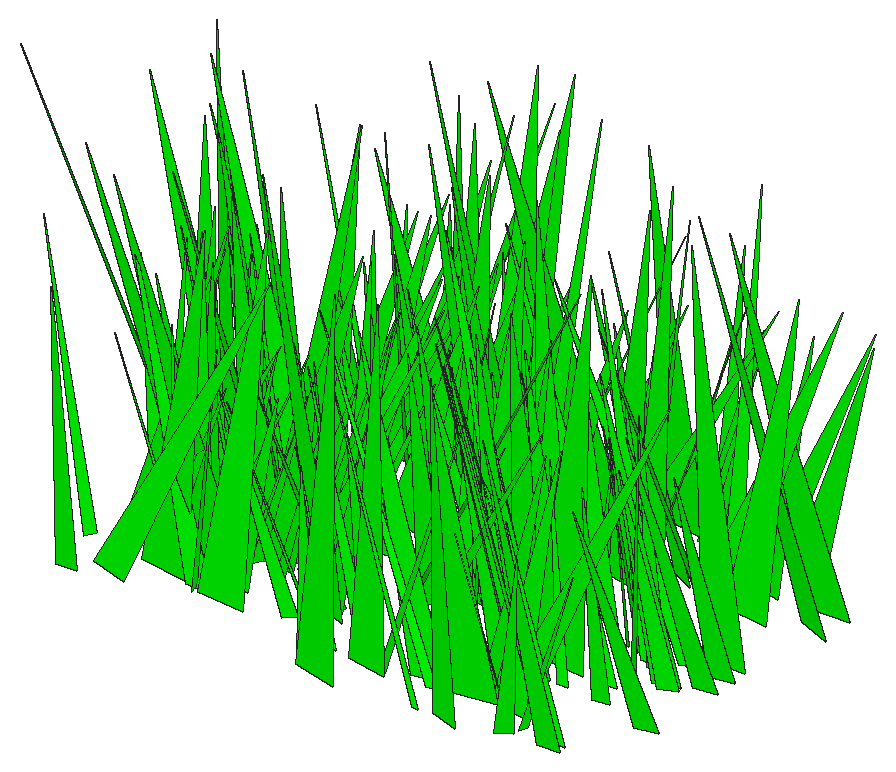
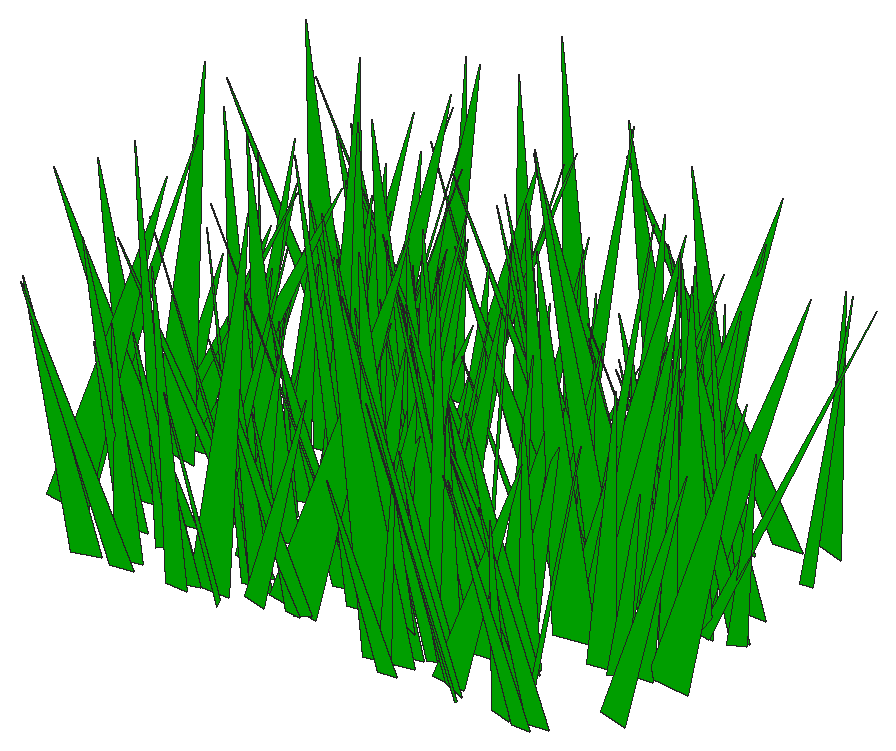
# SketchUp Ruby script. Lengths in inches.
U = 1.inch
M = Sketchup.active_model
def pt(a) = Geom::Point3d.new(a.map { |v| v * U })
def face(e, loops, mat)
  f = e.add_face(loops[0].map { |a| pt(a) })
  loops[1..].each { |l| e.add_face(l.map { |a| pt(a) }).erase! }
  f.material = f.back_material = mat if mat
  f
end
# faces: each face lists its corners as indices into pts; further lists are holes
def faces(e, pts, list, mat = nil) = list.each { |f| face(e, (f[0].is_a?(Array) ? f : [f]).map { |l| l.map { |i| pts[i] } }, mat) }
# xy, xz, yz: faces in a plane at the given z, y or x. An outline is a flat list of corners, or four numbers for a rectangle; further outlines are holes
def ring(l) = l.size == 4 ? [[l[0], l[1]], [l[2], l[1]], [l[2], l[3]], [l[0], l[3]]] : l.each_slice(2).to_a
def flat(e, list, mat, &to3) = list.each { |f| face(e, (f[0].is_a?(Array) ? f : [f]).map { |l| ring(l).map { |u, v| to3.(u, v) } }, mat) }
def xy(e, z, list, mat = nil) = flat(e, list, mat) { |x, y| [x, y, z] }
def xz(e, y, list, mat = nil) = flat(e, list, mat) { |x, z| [x, y, z] }
def yz(e, x, list, mat = nil) = flat(e, list, mat) { |y, z| [x, y, z] }
def lines(e, pts, list) = list.each { |a, b| e.add_line(pt(pts[a]), pt(pts[b])) }
# prism: a flat outline (further loops are holes) pulled along v
def prism(e, loops, v, mat = nil)
  f = face(e, loops, mat); d = Geom::Vector3d.new(v.map { |x| x * U })
  f.pushpull(f.normal.samedirection?(d) ? d.length : -d.length)
end
def box(e, o, s, mat = nil) = prism(e, [[o, [o[0] + s[0], o[1], o[2]], [o[0] + s[0], o[1] + s[1], o[2]], [o[0], o[1] + s[1], o[2]]]], [0, 0, s[2]], mat)
def at(x, y, z, deg = 0) = Geom::Transformation.translation(pt([x, y, z])) * Geom::Transformation.rotation(ORIGIN, Z_AXIS, deg.degrees)
def axes(o, x, y, z) = Geom::Transformation.new([*x, 0, *y, 0, *z, 0, *pt(o).to_a, 1])
def part(name) = M.definitions.add(name)
# library, detail: a bought-in or finely detailed component or shape, given as its bounding box
def library(name, o, s) = part(name).tap { |d| box(d.entities, o, s) }
def detail(e, o, s) = box(e.add_group.entities, o, s)
def put(e, d, t, mat = nil) = e.add_instance(d, t).tap { |i| i.material = mat if mat }
def group(e, t, mat = nil) = e.add_group.tap { |g| g.transformation = t; g.material = mat if mat }.entities
root = M.entities
M.materials.add("[0065_Lime]").color = [0, 255, 0]
c1 = part("fur_instance\#9")
p = [[0.8125,0,1.79],[0.67,-0.02,1.48],[0,-0.11,0],[0,0.11,0]]
faces(c1.entities,p,[[0,1,2,3]])
put(root,c1,axes([8.88,25.61,1.48],[-8.62925,-0.3961,0.13549],[2.79602,-1.20907,-0.62155],[0.39508,-0.09484,7.35796]),"[0065_Lime]")
put(root,c1,axes([7.83,28.66,1.48],[-2.89085,0.95849,0.65848],[-6.84022,-0.39041,-0.8262],[-0.62787,-0.15977,5.96919]),"[0065_Lime]")
put(root,c1,axes([7.84,31.3,1.48],[-3.93872,-0.61355,1.13712],[4.57864,-0.53971,0.73509],[0.23551,0.23156,4.72634]),"[0065_Lime]")
put(root,c1,axes([7.76,25.39,1.48],[-3.46221,0.44364,0.53192],[-3.06951,-0.4948,0.60947],[0.98674,0.01743,3.76228]),"[0065_Lime]")
put(root,c1,axes([8.42,21.2,1.48],[-6.26026,0.16791,1.68838],[-1.46894,-0.91389,-0.55815],[1.89171,-0.15397,5.15398]),"[0065_Lime]")
put(root,c1,axes([8.77,28.79,1.48],[-6.52964,0.43859,2.14545],[-3.49031,-0.96192,-0.43907],[2.12529,-0.23223,5.87052]),"[0065_Lime]")
put(root,c1,axes([8.57,27.79,1.48],[7.36202,0.5711,3.10917],[-4.17244,1.15392,-0.5655],[-3.70394,-0.16475,6.81686]),"[0065_Lime]")
put(root,c1,axes([10.42,24.13,1.48],[-4.90987,-0.85429,0.54019],[6.11505,-0.68391,0.53161],[-0.09449,0.13025,6.33426]),"[0065_Lime]")
put(root,c1,axes([9.12,19.1875,1.48],[3.68208,0.56895,1.86602],[-4.15905,0.58673,-0.56459],[-2.08778,-0.16541,4.4157]),"[0065_Lime]")
put(root,c1,axes([9.43,29.08,1.48],[-3.29767,0.49856,0.06601],[-3.46478,-0.45565,0.79286],[0.76819,0.08508,3.85945]),"[0065_Lime]")
put(root,c1,axes([10.11,32.61,1.48],[-6.0484,0.01018,1.35897],[-0.21877,-0.87821,-0.4237],[1.65791,-0.07873,4.90192]),"[0065_Lime]")
put(root,c1,axes([7.83,25.17,1.48],[4.07631,0.52223,1.15314],[-3.95918,0.56016,0.75946],[-0.383,-0.23238,4.4222]),"[0065_Lime]")
put(root,c1,axes([9.53,25.45,1.48],[1.71845,1.14041,0.61602],[-8.06483,0.25366,-0.84991],[-1.18209,-0.07274,6.69408]),"[0065_Lime]")
put(root,c1,axes([9.3125,23.78,1.48],[5.66093,-0.3191,1.47191],[2.11176,0.83483,0.69095],[-1.99297,-0.02181,4.91301]),"[0065_Lime]")
put(root,c1,axes([10.11,29.02,1.48],[-2.78205,-0.76326,0.72818],[5.37469,-0.40708,-0.71154],[1.19079,0.05417,4.9128]),"[0065_Lime]")
put(root,c1,axes([11.47,26.69,1.48],[2.49787,0.8466,3.05424],[-6.64063,0.4764,-0.83161],[-2.51001,-0.41788,5.23963]),"[0065_Lime]")
put(root,c1,axes([9.33,33.09,1.48],[2.13609,0.55662,0.59506],[-4.02276,0.28872,0.50476],[0.20946,-0.13155,3.62577]),"[0065_Lime]")
put(root,c1,axes([8.57,23.7,1.48],[6.07863,-0.66158,0.15927],[4.66708,0.85144,0.65963],[-0.65068,-0.07336,6.21923]),"[0065_Lime]")
put(root,c1,axes([10.14,24.2,1.48],[4.074,-0.8329,1.05894],[5.94379,0.59211,0.47582],[-1.22487,0.10294,5.83107]),"[0065_Lime]")
put(root,c1,axes([10.63,33.27,1.48],[2.79915,0.46696,0.77737],[-3.25281,0.4142,-0.58765],[-1.17287,-0.03432,3.48501]),"[0065_Lime]")
put(root,c1,axes([12.72,26.39,1.48],[-6.65494,0.87321,1.5159],[-6.43823,-0.93512,-0.65099],[0.79931,-0.26193,7.37763]),"[0065_Lime]")
put(root,c1,axes([10.52,25.25,1.48],[4.95752,0.29422,1.33139],[-1.861,0.73183,-0.83444],[-1.89736,0.05095,4.29717]),"[0065_Lime]")
put(root,c1,axes([12.44,20.97,1.48],[-4.88717,0.05899,0.36566],[-0.35143,-0.68297,0.58431],[0.50479,0.09564,3.94691]),"[0065_Lime]")
put(root,c1,axes([10.31,26.26,1.48],[-1.36301,-0.80322,0.96854],[5.6929,-0.22099,-0.84037],[1.29726,0.12586,4.70549]),"[0065_Lime]")
put(root,c1,axes([9.68,33.46,1.48],[3.58541,0.49358,0.56471],[-3.57861,0.49853,0.4321],[-0.11784,-0.12171,4.05984]),"[0065_Lime]")
put(root,c1,axes([12.33,25.76,1.48],[-5.36968,-0.09343,1.03645],[0.91105,-0.75686,0.83669],[1.11161,0.16897,4.32086]),"[0065_Lime]")
put(root,c1,axes([12.22,22.4,1.48],[-0.98241,-0.80155,1.19194],[5.85081,-0.10895,0.73554],[-0.67361,0.22268,4.65041]),"[0065_Lime]")
put(root,c1,axes([12.67,26.51,1.48],[-7.97788,-0.4692,2.19311],[3.70884,-1.15613,0.63841],[2.15946,0.25223,7.00575]),"[0065_Lime]")
put(root,c1,axes([11.4,22.58,1.48],[-3.01505,0.83014,1.46664],[-6.02476,-0.45741,0.48073],[1.36189,-0.18565,5.37361]),"[0065_Lime]")
put(root,c1,axes([12.68,23.37,1.48],[-6.42094,0.02711,1.19381],[-0.08857,-0.92342,0.38745],[1.47763,0.06245,5.21085]),"[0065_Lime]")
put(root,c1,axes([13.31,21.73,1.48],[-3.44753,-1.13548,0.28155],[8.0689,-0.47921,0.61174],[-0.55694,0.08607,7.11992]),"[0065_Lime]")
put(root,c1,axes([12.07,26.1875,1.48],[-5.60729,-0.01368,1.53159],[-0.25917,-0.81669,-0.87217],[1.86753,-0.1544,4.47758]),"[0065_Lime]")
put(root,c1,axes([13.07,20.65,1.48],[-6.38328,0.53031,0.68957],[-3.68099,-0.90345,0.73672],[1.18823,0.05009,5.98668]),"[0065_Lime]")
put(root,c1,axes([13.125,32.67,1.48],[-2.53373,0.72992,0.63177],[-5.2212,-0.33687,-0.81252],[-0.57049,-0.1587,4.63039]),"[0065_Lime]")
put(root,c1,axes([11.33,23.22,1.48],[-3.24539,-0.73169,1.37816],[5.18511,-0.49961,-0.80946],[1.76045,0.12264,4.92476]),"[0065_Lime]")
put(root,c1,axes([13.82,24.02,1.48],[-7.20391,-0.33541,0.88015],[2.50386,-1.01219,0.6342],[0.77399,0.15262,6.14038]),"[0065_Lime]")
put(root,c1,axes([9.87,24.01,1.48],[3.69943,0.42219,0.26454],[-3.00363,0.50568,0.74834],[0.33365,-0.12885,3.80367]),"[0065_Lime]")
put(root,c1,axes([11.7,21.29,1.48],[-4.86679,0.05739,1.93325],[-0.92596,-0.73901,-0.80718],[2.2267,-0.18188,3.88976]),"[0065_Lime]")
put(root,c1,axes([10.55,32.25,1.48],[3.71266,0.37883,0.38097],[-2.73631,0.51357,0.53104],[0.01046,-0.11289,3.69416]),"[0065_Lime]")
put(root,c1,axes([11.92,30.24,1.48],[3.69219,-0.52657,0.81287],[3.63765,0.53743,0.73356],[-1.34489,0.00802,4.21577]),"[0065_Lime]")
put(root,c1,axes([10.98,21.46,1.48],[3.51736,0.35367,0.72322],[-2.66268,0.47946,0.71149],[-0.18847,-0.17325,3.44541]),"[0065_Lime]")
put(root,c1,axes([11.56,20.87,1.48],[-0.43861,-1.06907,1.93122],[7.87846,-0.10863,-0.83123],[1.20398,0.3214,6.1428]),"[0065_Lime]")
put(root,c1,axes([11.76,28.23,1.48],[3.33834,-0.96689,2.25359],[7.39034,0.4702,-0.48339],[-0.63701,0.38797,6.20215]),"[0065_Lime]")
put(root,c1,axes([11.78,30.71,1.48],[0.18851,0.79547,0.50591],[-5.61388,0.01124,0.79169],[0.95821,-0.09063,4.53875]),"[0065_Lime]")
put(root,c1,axes([13.32,23.55,1.48],[2.37945,-1.02397,1.53397],[7.35764,0.37505,0.83788],[-1.58846,0.20335,6.17886]),"[0065_Lime]")
put(root,c1,axes([13.4,28.67,1.48],[-2.46533,-0.67082,0.0414],[4.74604,-0.34523,-0.45277],[0.51783,-0.02957,4.34689]),"[0065_Lime]")
put(root,c1,axes([12.29,23.29,1.48],[3.5173,0.46132,0.30432],[-3.19533,0.49443,-0.67979],[-0.84131,0.05078,3.85415]),"[0065_Lime]")
put(root,c1,axes([10.29,19.78,1.48],[5.55002,0.84243,0.01692],[-5.94926,0.7734,0.83715],[0.74123,-0.10037,6.59247]),"[0065_Lime]")
put(root,c1,axes([12.95,20.59,1.48],[-4.83925,-0.04488,2.25602],[-0.15329,-0.77445,-0.7338],[2.78764,-0.1205,3.87602]),"[0065_Lime]")
put(root,c1,axes([11.93,22.89,1.48],[4.97057,0.2584,0.09263],[-1.79018,0.68823,-0.77514],[-0.43579,0.12015,4.24069]),"[0065_Lime]")
put(root,c1,axes([13.63,31.9375,1.48],[-2.86629,-0.62619,1.39642],[4.53976,-0.4446,-0.51528],[1.48208,0.15082,4.27898]),"[0065_Lime]")
put(root,c1,axes([12.59,30.13,1.48],[1.72581,0.65738,0.09967],[-4.62875,0.23707,0.63439],[0.69004,-0.0539,4.00614]),"[0065_Lime]")
put(root,c1,axes([12.51,25.6875,1.48],[6.65704,0.81703,2.32683],[-6.32294,0.94512,0.84849],[-1.41818,-0.37861,7.13934]),"[0065_Lime]")
put(root,c1,axes([12.25,33.42,1.48],[5.83754,0.12789,0.64655],[-1.01532,0.81789,0.64412],[-0.6552,-0.12798,4.76234]),"[0065_Lime]")
put(root,c1,axes([12.5,29.53,1.48],[3.62361,-0.33149,0.10553],[2.34648,0.50104,-0.57099],[0.27589,0.09252,3.47043]),"[0065_Lime]")
put(root,c1,axes([14.53,27.91,1.48],[-2.95953,-0.69051,0.57175],[4.84112,-0.42691,-0.69685],[1.09794,0.02109,4.61376]),"[0065_Lime]")
put(root,c1,axes([13.36,32.26,1.48],[1.99452,0.52792,1.24768],[-4.05101,0.24492,0.81211],[0.23826,-0.25498,3.36324]),"[0065_Lime]")
put(root,c1,axes([13.43,23.02,1.48],[4.16785,-0.23891,0.29007],[1.61856,0.58134,0.65739],[-0.63105,-0.08686,3.60193]),"[0065_Lime]")
put(root,c1,axes([13.03,30.68,1.48],[3.16139,0.91934,1.09871],[-6.67484,0.42606,0.76153],[0.27463,-0.22769,5.86122]),"[0065_Lime]")
put(root,c1,axes([13.81,21.47,1.48],[1.29704,-0.56234,1.33332],[4.31055,0.14873,-0.67241],[0.34844,0.25327,3.3552]),"[0065_Lime]")
put(root,c1,axes([12.74,32.89,1.48],[7.40801,0.50292,0.72367],[-3.49787,1.04704,-0.6915],[-1.16876,0.0541,6.65636]),"[0065_Lime]")
put(root,c1,axes([15.33,28.08,1.48],[-7.49179,-0.15952,2.36966],[1.42562,-1.12024,0.45517],[2.78267,0.14445,6.14665]),"[0065_Lime]")
put(root,c1,axes([14.97,23.92,1.48],[2.78676,-0.42596,1.13511],[2.99621,0.43186,0.56347],[-1.46945,0.07274,3.30163]),"[0065_Lime]")
put(root,c1,axes([14.93,30.875,1.48],[-5.96306,-0.60382,3.06183],[5.06929,-0.91181,0.50671],[2.6337,0.38791,5.95711]),"[0065_Lime]")
put(root,c1,axes([14.08,20.43,1.48],[-3.26996,0.99545,2.59711],[-7.38667,-0.5493,0.90155],[2.41185,-0.3327,6.28225]),"[0065_Lime]")
put(root,c1,axes([16.34,20.98,1.48],[-3.97649,0.2994,0.68303],[-2.2721,-0.54541,-0.74081],[0.28738,-0.16932,3.59404]),"[0065_Lime]")
put(root,c1,axes([16.07,25.79,1.48],[-0.33969,0.67541,0.22034],[-4.70442,-0.03847,-0.84754],[-1.02236,-0.04741,3.82677]),"[0065_Lime]")
put(root,c1,axes([15.96,23.8,1.48],[-3.69634,-0.3812,1.09806],[2.94626,-0.52205,0.48915],[0.70799,0.18228,3.69729]),"[0065_Lime]")
put(root,c1,axes([15.31,33.04,1.48],[-3.32047,-0.37518,1.07575],[2.63247,-0.49974,-0.46401],[1.39566,0.05,3.43457]),"[0065_Lime]")
put(root,c1,axes([14.2,31.88,1.48],[3.43404,-0.44583,0.64394],[3.26697,0.47475,-0.51309],[-0.142,0.14083,3.76824]),"[0065_Lime]")
put(root,c1,axes([17.21,20.98,1.48],[-4.46572,0.01531,0.0675],[-0.09671,-0.62186,0.49294],[0.09698,0.08486,3.59997]),"[0065_Lime]")
put(root,c1,axes([16.6,22.5,1.48],[6.26715,0.54743,4.3486],[-5.21873,1.04506,0.56792],[-4.06484,-0.49771,5.97551]),"[0065_Lime]")
put(root,c1,axes([13.95,30.46,1.48],[7.64694,0.51855,1.2893],[-3.63876,1.09725,-0.50857],[-1.70007,-0.01605,6.8878]),"[0065_Lime]")
put(root,c1,axes([17.24,22.39,1.48],[-3.8742,-0.23866,0.2948],[1.73257,-0.52259,0.88831],[-0.11941,0.16081,3.32421]),"[0065_Lime]")
put(root,c1,axes([14.35,23.75,1.48],[2.61119,-0.52349,0.68709],[3.81528,0.35023,-0.65201],[0.19037,0.16143,3.64269]),"[0065_Lime]")
put(root,c1,axes([15.27,23.3,1.48],[2.66129,-0.51278,0.27779],[3.5647,0.37592,0.65679],[-0.85224,-0.0289,3.61464]),"[0065_Lime]")
put(root,c1,axes([14.65,22.6,1.48],[4.3971,0.21892,0.90868],[-1.74515,0.61967,0.5848],[-0.7935,-0.14972,3.74919]),"[0065_Lime]")
put(root,c1,axes([13.81,23.21,1.48],[3.79893,-1.02081,0.57984],[7.28059,0.52176,-0.78026],[0.52518,0.15085,6.62252]),"[0065_Lime]")
put(root,c1,axes([14.61,24.28,1.48],[4.74162,-0.26585,0.30869],[1.81737,0.66281,0.65784],[-0.64857,-0.08633,4.10015]),"[0065_Lime]")
put(root,c1,axes([14.9,33.42,1.48],[2.02079,0.49789,0.2619],[-3.54744,0.27798,0.402],[0.2723,-0.07352,3.29348]),"[0065_Lime]")
put(root,c1,axes([16.03,29.8125,1.48],[2.45456,1.11267,1.01398],[-7.92955,0.36386,-0.67906],[-1.17357,-0.13134,6.70901]),"[0065_Lime]")
put(root,c1,axes([15.25,29.625,1.48],[5.79663,0.16091,1.31269],[-0.92894,0.84105,-0.74047],[-1.74718,0.08666,4.74879]),"[0065_Lime]")
put(root,c1,axes([15.76,32.13,1.48],[-1.07115,1.27684,0.81476],[-9.10381,-0.16188,0.58187],[0.83157,-0.12752,7.41961]),"[0065_Lime]")
put(root,c1,axes([18.09,30.08,1.48],[-8.06784,-0.58151,1.86564],[4.42615,-1.15273,0.62454],[1.67199,0.24559,7.34897]),"[0065_Lime]")
put(root,c1,axes([15.84,28.04,1.48],[3.88166,0.07753,0.99446],[-0.75201,0.56135,0.47565],[-1.11067,-0.10912,3.15346]),"[0065_Lime]")
put(root,c1,axes([17.3,27.2,1.48],[-2.28046,-0.76224,1.41769],[5.69726,-0.30809,0.51293],[0.06528,0.26028,4.75887]),"[0065_Lime]")
put(root,c1,axes([14.54,25.16,1.48],[2.82797,0.922,0.01793],[-6.50651,0.39361,0.75841],[0.84759,-0.05468,5.76208]),"[0065_Lime]")
put(root,c1,axes([15.13,25.76,1.48],[3.88426,0.28332,0.32782],[-2.05345,0.54071,0.43908],[-0.10522,-0.0935,3.53263]),"[0065_Lime]")
put(root,c1,axes([15.25,32.23,1.48],[4.38709,-0.92302,1.4892],[6.80457,0.6125,-0.54204],[-0.44436,0.26656,6.40225]),"[0065_Lime]")
put(root,c1,axes([16.14,24.31,1.48],[5.50877,-0.63428,1.36656],[4.41616,0.80832,0.79312],[-1.92221,0.03933,5.73849]),"[0065_Lime]")
put(root,c1,axes([15.81,30.11,1.48],[3.92881,-1.04232,0.03686],[7.3722,0.54946,0.7371],[-0.82189,-0.05401,6.78784]),"[0065_Lime]")
put(root,c1,axes([17.77,28.74,1.48],[-5.97453,-0.68617,1.93347],[5.22264,-0.8621,0.42564],[1.48972,0.27046,6.26203]),"[0065_Lime]")
put(root,c1,axes([15.31,32.84,1.48],[2.6676,-1.20208,1.85989],[8.84586,0.34656,-0.88886],[0.40104,0.35162,7.23453]),"[0065_Lime]")
put(root,c1,axes([15.35,27.55,1.48],[2.54463,0.74766,0.76131],[-5.38569,0.33963,0.73394],[0.42512,-0.17264,4.74098]),"[0065_Lime]")
put(root,c1,axes([16.25,28.02,1.48],[-3.03443,0.46201,1.43815],[-3.15952,-0.48836,0.84637],[1.98841,-0.07094,3.53956]),"[0065_Lime]")
put(root,c1,axes([17.4,21.82,1.48],[-4.31895,-0.46803,1.19725],[3.24184,-0.64032,-0.65019],[1.65857,0.03282,4.38854]),"[0065_Lime]")
put(root,c1,axes([15.73,23.62,1.48],[6.60703,-0.20696,0.88588],[1.29833,0.93317,0.89853],[-1.29219,-0.1206,5.43235]),"[0065_Lime]")
put(root,c1,axes([18.3,26.52,1.48],[-5.44796,0.14857,0.99663],[-0.91467,-0.78145,0.59543],[1.33511,0.07089,4.47468]),"[0065_Lime]")
put(root,c1,axes([15.1,23.27,1.48],[6.63846,0.45789,0.47369],[-3.30982,0.92099,0.85816],[-0.0511,-0.16918,5.95374]),"[0065_Lime]")
put(root,c1,axes([19.73,31.97,1.48],[-3.60052,-1.19561,0.63591],[8.52493,-0.49461,0.77482],[-0.57734,0.15298,7.47512]),"[0065_Lime]")
put(root,c1,axes([18.6,20.28,1.48],[-4.00301,0.07438,0.6728],[-0.39455,-0.56854,0.5529],[0.89924,0.08164,3.23757]),"[0065_Lime]")
put(root,c1,axes([19.03,28.44,1.48],[-5.33529,-0.65046,1.87881],[5.06284,-0.75233,0.7847],[1.06315,0.31843,5.6917]),"[0065_Lime]")
put(root,c1,axes([16.82,27.9,1.48],[5.58791,0.03082,1.13912],[-0.48943,0.79304,0.86953],[-1.33032,-0.16231,4.4649]),"[0065_Lime]")
put(root,c1,axes([18.35,19.34,1.48],[1.361,0.5669,0.27902],[-3.92791,0.1972,-0.74919],[-0.9826,-0.00309,3.38133]),"[0065_Lime]")
put(root,c1,axes([16.97,22.27,1.48],[5.1113,0.51565,1.43914],[-3.93248,0.72868,0.49216],[-1.064,-0.21606,5.09442]),"[0065_Lime]")
put(root,c1,axes([19.14,21.06,1.48],[-5.27029,0.23028,1.22832],[-1.86031,-0.75461,-0.54061],[1.22688,-0.155,4.45672]),"[0065_Lime]")
put(root,c1,axes([18.67,27.4,1.48],[2.27917,0.5778,1.02759],[-4.0396,0.35653,-0.78954],[-1.47832,-0.08345,3.74172]),"[0065_Lime]")
put(root,c1,axes([18.75,21.85,1.48],[1.72126,-0.50421,1.16046],[3.66858,0.28203,0.50584],[-1.2051,0.13838,3.19738]),"[0065_Lime]")
put(root,c1,axes([19.09,26.16,1.48],[-3.62573,-0.26441,1.4442],[2.26996,-0.53119,0.51181],[1.24106,0.19912,3.28307]),"[0065_Lime]")
put(root,c1,axes([20.43,30.36,1.48],[-6.01193,0.26272,1.11163],[-2.09546,-0.84457,-0.80953],[0.98614,-0.19296,5.05683]),"[0065_Lime]")
put(root,c1,axes([19.28,24.29,1.48],[1.39097,-0.7797,0.60209],[5.51249,0.20943,0.6619],[-0.97404,0.07183,4.60575]),"[0065_Lime]")
put(root,c1,axes([18.18,30.79,1.48],[8.58966,-0.39152,1.91768],[2.72544,1.25148,0.48462],[-2.42765,0.01969,7.32933]),"[0065_Lime]")
put(root,c1,axes([21.04,25.03,1.48],[-3.31148,0.50401,0.44402],[-3.6263,-0.45655,-0.52873],[-0.11358,-0.1182,3.93547]),"[0065_Lime]")
put(root,c1,axes([19.15,18.65,1.48],[4.90653,0.82522,3.29044],[-6.93491,0.7129,0.85092],[-1.66122,-0.53873,6.16632]),"[0065_Lime]")
put(root,c1,axes([20.83,32.44,1.48],[-3.29325,-0.47966,1.02887],[3.61804,-0.45776,0.51123],[0.40236,0.19025,3.82413]),"[0065_Lime]")
put(root,c1,axes([20.71,26.59,1.48],[-0.40222,0.64872,0.28326],[-4.5928,-0.04972,-0.49954],[-0.58357,-0.05583,3.73619]),"[0065_Lime]")
put(root,c1,axes([18.6,24.66,1.48],[3.5045,0.30337,0.17384],[-2.16669,0.48653,0.44933],[0.10981,-0.08179,3.31782]),"[0065_Lime]")
put(root,c1,axes([22.42,20.24,1.48],[-7.41794,0.17142,0.60519],[-1.1605,-1.04522,0.509],[0.83365,0.07028,6.09367]),"[0065_Lime]")
put(root,c1,axes([19.14,26.23,1.48],[4.77261,-0.13797,0.69381],[0.8116,0.67213,0.78495],[-1.01634,-0.11117,3.8849]),"[0065_Lime]")
put(root,c1,axes([20.06,20.03,1.48],[-3.90987,-0.89662,2.46447],[6.7444,-0.6185,-0.46072],[2.09946,0.31711,6.06968]),"[0065_Lime]")
put(root,c1,axes([19.46,32.29,1.48],[3.5945,-0.30436,0.20883],[2.10334,0.5021,0.56711],[-0.57735,-0.06571,3.36617]),"[0065_Lime]")
put(root,c1,axes([22.01,20.62,1.48],[-4.07292,0.8035,0.78333],[-5.79634,-0.56884,-0.38844],[0.1648,-0.14926,5.69726]),"[0065_Lime]")
put(root,c1,axes([19.21,30.04,1.48],[2.75632,0.66939,0.93001],[-4.88671,0.36259,0.83725],[0.34744,-0.21059,4.39779]),"[0065_Lime]")
put(root,c1,axes([20.59,23.92,1.48],[4.35814,-0.40503,2.03659],[3.39463,0.65543,-0.43841],[-1.74748,0.26309,4.2275]),"[0065_Lime]")
put(root,c1,axes([21.73,27.43,1.48],[-4.08363,-0.18354,1.03595],[1.60197,-0.57069,0.79001],[0.87284,0.18871,3.3968]),"[0065_Lime]")
put(root,c1,axes([19.15,32.21,1.48],[4.86568,-0.36094,0.34656],[2.60061,0.67989,-0.43062],[-0.12714,0.0938,4.45469]),"[0065_Lime]")
put(root,c1,axes([20.73,25.57,1.48],[3.89391,-0.58771,1.09593],[4.17824,0.57353,0.48374],[-1.3603,0.07931,4.623]),"[0065_Lime]")
put(root,c1,axes([20.55,26.41,1.48],[3.35078,-0.37271,1.48405],[3.08989,0.4762,-0.60843],[-0.90366,0.24627,3.42248]),"[0065_Lime]")
put(root,c1,axes([22.8,18.97,1.48],[-6.3911,0.06487,0.78103],[-0.34028,-0.90185,0.66758],[1.0096,0.10667,5.16922]),"[0065_Lime]")
put(root,c1,axes([20.66,25.18,1.48],[1.45123,1.05923,2.52911],[-8.15327,0.18211,0.53973],[0.11739,-0.44644,6.22077]),"[0065_Lime]")
put(root,c1,axes([18.74,30.05,1.48],[7.89936,0.16983,0.33747],[-1.14453,1.10269,-0.86923],[-0.56826,0.13989,6.44184]),"[0065_Lime]")
put(root,c1,axes([21.02,31.86,1.48],[4.78252,-0.34672,1.95755],[3.07805,0.6899,-0.88092],[-1.55101,0.30003,4.28785]),"[0065_Lime]")
put(root,c1,axes([21.5,23.46,1.48],[4.31571,0.19305,1.37628],[-1.11559,0.64875,-0.73465],[-1.87233,0.05843,3.61004]),"[0065_Lime]")
put(root,c1,axes([22.38,32.71,1.48],[-4.15673,-1.02032,1.30332],[7.32319,-0.60646,-0.45594],[1.28955,0.15512,6.79036]),"[0065_Lime]")
put(root,c1,axes([18.68,23.84,1.48],[8.80351,0.0353,0.26575],[-0.23274,1.23603,-0.40086],[-0.34014,0.06796,7.15258]),"[0065_Lime]")
put(root,c1,axes([22.54,30.55,1.48],[-0.51592,-0.67192,1.10329],[4.95474,-0.05433,0.42431],[-0.39422,0.19655,3.88903]),"[0065_Lime]")
put(root,c1,axes([20.65,20.01,1.48],[6.04736,0.29074,0.66619],[-1.94378,0.8524,-0.79106],[-1.08328,0.09353,5.13841]),"[0065_Lime]")
put(root,c1,axes([22.21,25.54,1.48],[-6.0089,0.6956,2.42363],[-5.10335,-0.9222,0.49752],[2.70901,-0.19437,6.31314]),"[0065_Lime]")
put(root,c1,axes([24.06,23.22,1.48],[-6.98863,-0.20797,0.81583],[1.37336,-0.98855,-0.66037],[1.14471,-0.08369,5.77308]),"[0065_Lime]")
put(root,c1,axes([24.19,22.75,1.48],[-7.33683,0.76233,0.72533],[-5.35594,-1.03821,0.71882],[1.24153,0.02617,7.38732]),"[0065_Lime]")
put(root,c1,axes([23.63,22.51,1.48],[-1.54999,0.82446,0.86921],[-5.91675,-0.19313,-0.84242],[-0.74779,-0.18079,4.86385]),"[0065_Lime]")
put(root,c1,axes([23.85,24.06,1.48],[-4.08994,0.04752,0.22068],[-0.39168,-0.56005,-0.76175],[0.1859,-0.13449,3.25009]),"[0065_Lime]")
put(root,c1,axes([22.59,24.99,1.48],[0.93365,-1.02712,0.56624],[7.31694,0.13839,0.42915],[-0.61364,0.08735,5.97861]),"[0065_Lime]")
put(root,c1,axes([21.53,25.33,1.48],[5.52747,-0.54721,0.84851],[3.75249,0.78926,0.88226],[-1.4738,-0.04274,5.42868]),"[0065_Lime]")
put(root,c1,axes([23.1,23.12,1.48],[0.97161,-0.92558,1.68196],[6.82649,0.17261,0.57382],[-1.03083,0.27068,5.3854]),"[0065_Lime]")
put(root,c1,axes([21.65,33.17,1.48],[4.35714,0.01412,0.74447],[0.11291,0.60915,-0.82442],[-0.91379,0.1426,3.4479]),"[0065_Lime]")
put(root,c1,axes([21.79,31.6875,1.48],[7.01965,-0.0943,1.78893],[0.46903,1.03062,0.60267],[-2.25104,-0.07932,5.70416]),"[0065_Lime]")
put(root,c1,axes([20.39,22.17,1.48],[5.92617,-0.21926,0.14172],[1.57008,0.8278,-0.52394],[-0.00347,0.09376,4.95711]),"[0065_Lime]")
put(root,c1,axes([24.35,22.7,1.48],[-2.16815,0.87427,0.44271],[-6.21778,-0.29453,-0.65744],[-0.58809,-0.10917,5.31887]),"[0065_Lime]")
put(root,c1,axes([24.18,30.19,1.48],[-6.05276,-0.49832,0.83255],[3.41893,-0.86102,-0.82332],[1.39097,-0.05207,5.6465]),"[0065_Lime]")
put(root,c1,axes([23.79,20.57,1.48],[0.22039,-1.17281,0.73334],[8.33619,0.04554,0.78276],[-0.99121,0.12221,6.74614]),"[0065_Lime]")
put(root,c1,axes([23.3,25.14,1.48],[-6.14493,0.81191,3.37158],[-6.66719,-0.92551,-0.57167],[2.47279,-0.47776,6.8371]),"[0065_Lime]")
put(root,c1,axes([24.77,21.58,1.48],[-6.88948,-0.13973,1.13089],[1.1407,-0.98005,0.54014],[1.27303,0.12196,5.63625]),"[0065_Lime]")
put(root,c1,axes([23.87,26.75,1.48],[-3.45394,0.66845,0.44516],[-4.72032,-0.49124,0.48511],[0.80457,-0.01246,4.75713]),"[0065_Lime]")
put(root,c1,axes([24.04,24.42,1.48],[2.4702,-0.696,2.3908],[5.44603,0.4285,0.45707],[-1.87433,0.32779,4.47891]),"[0065_Lime]")
put(root,c1,axes([22.65,29,1.48],[-2.84255,-1.04223,2.44475],[7.72363,-0.47464,-0.83862],[2.0958,0.33559,6.4064]),"[0065_Lime]")
put(root,c1,axes([23.35,27.37,1.48],[3.55477,0.25805,1.00402],[-1.72989,0.52876,-0.50152],[-1.37968,0.0019,3.21568]),"[0065_Lime]")
put(root,c1,axes([22.46,24.89,1.48],[3.69201,0.62017,1.25484],[-4.65431,0.5137,0.55322],[-0.44281,-0.22859,4.64766]),"[0065_Lime]")
put(root,c1,axes([23.96,18.9,1.48],[5.36662,0.52323,3.00878],[-4.56475,0.83219,0.53762],[-2.59046,-0.38247,5.28587]),"[0065_Lime]")
put(root,c1,axes([23.25,33.1875,1.48],[5.74009,-0.43556,1.39991],[2.97877,0.84205,0.69776],[-1.92274,0.00422,5.26026]),"[0065_Lime]")
put(root,c1,axes([24.875,20.67,1.48],[-3.97241,-0.13486,0.47585],[0.81336,-0.55329,-0.76208],[0.77577,-0.11048,3.23565]),"[0065_Lime]")
put(root,c1,axes([23.05,32.87,1.48],[2.87306,-0.57191,0.95212],[4.23479,0.3901,-0.60287],[-0.04553,0.19457,4.00729]),"[0065_Lime]")
put(root,c1,axes([23.21,32.35,1.48],[4.28471,-0.11405,0.79682],[0.99965,0.60096,-0.67436],[-0.7868,0.14246,3.48252]),"[0065_Lime]")
put(root,c1,axes([21.5625,31,1.48],[5.63441,0.55056,0.06642],[-3.88039,0.78096,0.87571],[0.54847,-0.13068,5.51319]),"[0065_Lime]")
put(root,c1,axes([24,28.625,1.48],[5.68736,0.9446,1.95902],[-6.80328,0.84822,-0.63673],[-2.16896,-0.18368,7.13405]),"[0065_Lime]")
put(root,c1,axes([26.74,20.21,1.48],[-7.24798,0.00168,0.88209],[0.09009,-1.02525,0.55515],[1.08075,0.09672,5.86941]),"[0065_Lime]")
put(root,c1,axes([23.05,29.91,1.48],[6.72118,0.0891,0.76098],[-0.50727,0.94626,-0.748],[-1.00992,0.11764,5.44019]),"[0065_Lime]")
put(root,c1,axes([27.79,26.21,1.48],[-6.51766,0.58567,0.10081],[-4.16547,-0.91301,-0.4446],[-0.19037,-0.07407,6.27716]),"[0065_Lime]")
put(root,c1,axes([25.43,25.98,1.48],[-4.06448,-0.07977,1.21829],[0.78786,-0.59935,0.42409],[1.39456,0.10612,3.31115]),"[0065_Lime]")
put(root,c1,axes([25.58,27.05,1.48],[3.41253,-0.4015,1.8181],[2.93422,0.55905,0.49297],[-2.13316,0.12669,3.58661]),"[0065_Lime]")
put(root,c1,axes([25.92,25.93,1.48],[-4.39779,-0.08793,1.05584],[0.94683,-0.61791,0.88491],[1.08629,0.18259,3.50322]),"[0065_Lime]")
put(root,c1,axes([25.42,22.82,1.48],[-4.26066,0.21881,1.21854],[-1.46651,-0.63463,0.42596],[1.58693,0.00101,3.66522]),"[0065_Lime]")
put(root,c1,axes([24.01,21.22,1.48],[4.97533,-0.57124,0.19568],[3.98788,0.69424,0.8239],[-0.8253,-0.08917,5.16081]),"[0065_Lime]")
put(root,c1,axes([24.47,23.76,1.48],[1.02011,-1.24955,1.63724],[9.10361,0.12394,-0.58337],[0.50165,0.29186,7.25728]),"[0065_Lime]")
put(root,c1,axes([26.6,23.72,1.48],[-4.20532,0.23426,0.49979],[-1.60721,-0.59613,0.41543],[0.75749,0.03571,3.65613]),"[0065_Lime]")
put(root,c1,axes([26.77,25.57,1.48],[-6.5527,0.54879,1.20034],[-3.83277,-0.94374,0.61469],[1.65544,-0.01273,6.17443]),"[0065_Lime]")
put(root,c1,axes([25.1,31.44,1.48],[-7.36746,0.33276,3.17213],[-2.3152,-1.16953,0.55324],[3.9314,-0.06515,6.27039]),"[0065_Lime]")
put(root,c1,axes([25.08,20.64,1.48],[0.84583,0.83957,0.8093],[-6.03119,0.1037,0.56594],[0.55967,-0.15139,4.87573]),"[0065_Lime]")
put(root,c1,axes([25.4,32.83,1.48],[-0.7216,-0.72555,0.14823],[5.07877,-0.10436,-0.75838],[0.94875,0.00681,4.17244]),"[0065_Lime]")
put(root,c1,axes([25.5,32.55,1.48],[3.0979,-0.40093,1.04451],[3.07374,0.43742,-0.40551],[-0.58481,0.17525,3.40172]),"[0065_Lime]")
put(root,c1,axes([27.5,19.55,1.48],[-4.24879,-0.61153,1.32981],[4.6163,-0.59177,0.6398],[0.54968,0.24295,4.90571]),"[0065_Lime]")
put(root,c1,axes([25.875,19.44,1.48],[3.12118,-0.47583,0.11657],[3.26957,0.42992,0.88278],[-0.89278,-0.08902,3.64047]),"[0065_Lime]")
put(root,c1,axes([27.51,19.94,1.48],[-3.72174,0.38067,0.07652],[-2.67993,-0.5201,0.45824],[0.40709,0.05629,3.71623]),"[0065_Lime]")
put(root,c1,axes([26.96,22.78,1.48],[2.24545,0.50759,1.17186],[-3.57335,0.36154,-0.71721],[-1.53468,-0.09914,3.38454]),"[0065_Lime]")
put(root,c1,axes([27.88,24.8,1.48],[2.9369,-0.57027,3.10145],[4.77955,0.56896,0.51102],[-2.8573,0.36558,4.04266]),"[0065_Lime]")
put(root,c1,axes([29.23,26.27,1.48],[-6.69354,-0.28533,0.34812],[2.06898,-0.93328,0.68851],[0.16035,0.13136,5.64782]),"[0065_Lime]")
put(root,c1,axes([26.93,25.52,1.48],[-3.98999,0.3439,1.9552],[-3.0631,-0.59042,-0.65597],[1.54432,-0.28255,3.75048]),"[0065_Lime]")
put(root,c1,axes([24.31,22.53,1.48],[5.56273,0.70799,0.1491],[-5.02733,0.776,0.62579],[0.38148,-0.09735,6.07277]),"[0065_Lime]")
put(root,c1,axes([28.09,24.62,1.48],[-2.74512,0.46745,0.89348],[-3.50029,-0.37407,-0.55767],[0.14456,-0.18081,3.46365]),"[0065_Lime]")
put(root,c1,axes([25.28,33.31,1.48],[3.76018,0.62923,0.43375],[-4.49387,0.51471,0.75561],[0.37579,-0.14094,4.69585]),"[0065_Lime]")
put(root,c1,axes([26.18,20,1.48],[3.94277,-0.15701,0.3316],[1.03357,0.55043,0.60193],[-0.58853,-0.08518,3.2786]),"[0065_Lime]")
put(root,c1,axes([29.28,30.21,1.48],[-7.28856,-0.71993,0.56151],[5.04469,-1.0271,-0.80216],[1.1301,-0.05827,7.20227]),"[0065_Lime]")
put(root,c1,axes([29.05,31.27,1.48],[-3.4459,-1.03845,0.61916],[7.4211,-0.47559,0.59814],[-0.34899,0.1404,6.60563]),"[0065_Lime]")
put(root,c1,axes([27.42,23.78,1.48],[5.36372,0.22285,1.8645],[-1.40761,0.81945,-0.60269],[-2.4058,0.01738,4.50953]),"[0065_Lime]")
put(root,c1,axes([26.51,31.21,1.48],[2.74906,0.70445,1.53923],[-5.35561,0.37099,0.6393],[-0.17532,-0.28687,4.60654]),"[0065_Lime]")
put(root,c1,axes([29.01,25.27,1.48],[-2.24919,-0.66379,0.52736],[4.73348,-0.2987,0.75871],[-0.57436,0.13771,4.18763]),"[0065_Lime]")
put(root,c1,axes([28.49,26.82,1.48],[-4.13246,-0.98157,2.89725],[7.75638,-0.59466,0.56888],[1.14945,0.48381,6.5773]),"[0065_Lime]")
put(root,c1,axes([25.68,30.05,1.48],[3.25957,0.97482,0.10204],[-6.87351,0.451,0.89867],[0.94728,-0.08182,6.16967]),"[0065_Lime]")
put(root,c1,axes([29.125,22.27,1.48],[-1.12309,-0.65138,0.13586],[4.55444,-0.15027,0.76783],[-0.87943,0.05361,3.80298]),"[0065_Lime]")
put(root,c1,axes([27.09,29.63,1.48],[0.9525,0.99248,1.49064],[-7.27379,0.10848,0.65495],[0.58058,-0.26918,5.76008]),"[0065_Lime]")
put(root,c1,axes([26.64,33.33,1.48],[1.74228,-0.74856,0.73118],[5.35231,0.22112,-0.85263],[0.73451,0.16431,4.47862]),"[0065_Lime]")
put(root,c1,axes([28.96,26.12,1.48],[-0.33193,-0.65556,0.01956],[4.62128,-0.04574,0.5231],[-0.63979,0.00975,3.76827]),"[0065_Lime]")
